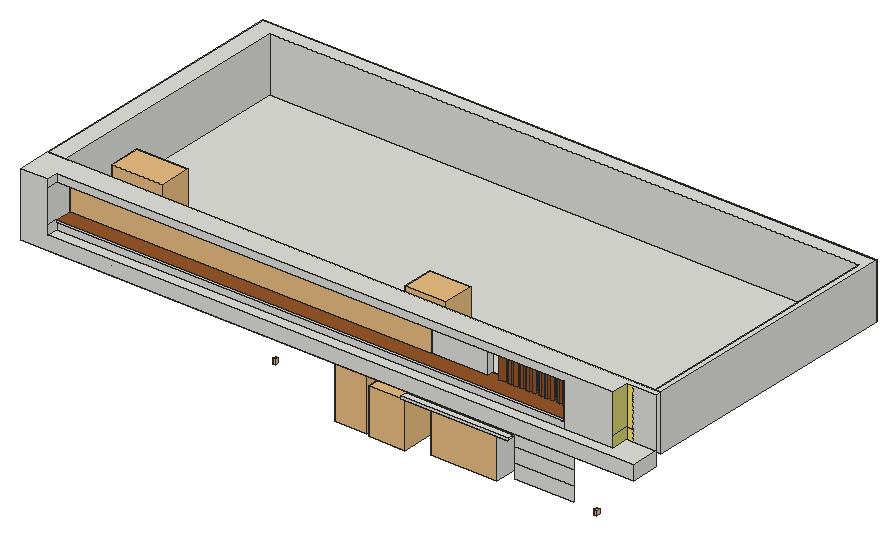
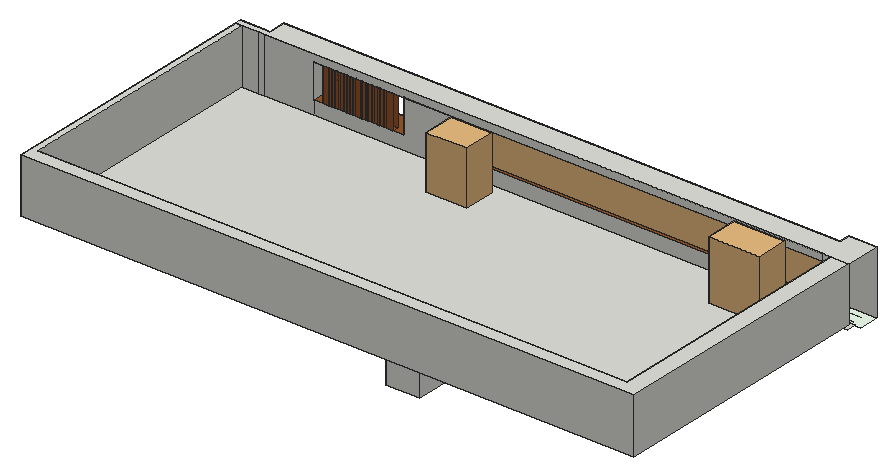
# SketchUp Ruby script. Lengths in inches.
U = 1.inch
M = Sketchup.active_model
def pt(a) = Geom::Point3d.new(a.map { |v| v * U })
def face(e, loops, mat)
  f = e.add_face(loops[0].map { |a| pt(a) })
  loops[1..].each { |l| e.add_face(l.map { |a| pt(a) }).erase! }
  f.material = f.back_material = mat if mat
  f
end
# faces: each face lists its corners as indices into pts; further lists are holes
def faces(e, pts, list, mat = nil) = list.each { |f| face(e, (f[0].is_a?(Array) ? f : [f]).map { |l| l.map { |i| pts[i] } }, mat) }
# xy, xz, yz: faces in a plane at the given z, y or x. An outline is a flat list of corners, or four numbers for a rectangle; further outlines are holes
def ring(l) = l.size == 4 ? [[l[0], l[1]], [l[2], l[1]], [l[2], l[3]], [l[0], l[3]]] : l.each_slice(2).to_a
def flat(e, list, mat, &to3) = list.each { |f| face(e, (f[0].is_a?(Array) ? f : [f]).map { |l| ring(l).map { |u, v| to3.(u, v) } }, mat) }
def xy(e, z, list, mat = nil) = flat(e, list, mat) { |x, y| [x, y, z] }
def xz(e, y, list, mat = nil) = flat(e, list, mat) { |x, z| [x, y, z] }
def yz(e, x, list, mat = nil) = flat(e, list, mat) { |y, z| [x, y, z] }
def lines(e, pts, list) = list.each { |a, b| e.add_line(pt(pts[a]), pt(pts[b])) }
# prism: a flat outline (further loops are holes) pulled along v
def prism(e, loops, v, mat = nil)
  f = face(e, loops, mat); d = Geom::Vector3d.new(v.map { |x| x * U })
  f.pushpull(f.normal.samedirection?(d) ? d.length : -d.length)
end
def box(e, o, s, mat = nil) = prism(e, [[o, [o[0] + s[0], o[1], o[2]], [o[0] + s[0], o[1] + s[1], o[2]], [o[0], o[1] + s[1], o[2]]]], [0, 0, s[2]], mat)
def at(x, y, z, deg = 0) = Geom::Transformation.translation(pt([x, y, z])) * Geom::Transformation.rotation(ORIGIN, Z_AXIS, deg.degrees)
def axes(o, x, y, z) = Geom::Transformation.new([*x, 0, *y, 0, *z, 0, *pt(o).to_a, 1])
def part(name) = M.definitions.add(name)
# library, detail: a bought-in or finely detailed component or shape, given as its bounding box
def library(name, o, s) = part(name).tap { |d| box(d.entities, o, s) }
def detail(e, o, s) = box(e.add_group.entities, o, s)
def put(e, d, t, mat = nil) = e.add_instance(d, t).tap { |i| i.material = mat if mat }
def group(e, t, mat = nil) = e.add_group.tap { |g| g.transformation = t; g.material = mat if mat }.entities
root = M.entities
M.materials.add("Emissive").color = [210, 207, 113]
M.materials.add("Generic").color = [255, 233, 107]
M.materials.add("[0066_Honeydew]").color = [240, 255, 240]
M.materials.add("[Wood Cherry Original]").color = [152, 86, 42]
M.materials.add("[Wood Veneer 01]").color = [120, 70, 37]
c1 = library("KentiaPalm",[-22.86,-14.31,0],[47.49,43.96,59.125])
c2 = library("cay+chuoi",[26.89,19.66,0.52],[41.96,45.65,69.71])
c3 = library("Group\#14",[0,0,0],[39.5,117.4375,51.17])
c4 = part("Group668\#1")
p = [[0,0,0],[0,0,-13.34],[-3.03,0,-13.34],[19.7,-23.5,0],[-19.7,-23.5,0],[19.7,23.5,0],
  [19.7,0,0],[-19.7,23.5,0],[3.03,0,-13.34],[-19.7,0,0],[0,0,-21.6]]
lines(c4.entities,p,[[0,1],[1,2],[3,4],[5,6],[7,5],[1,8],[9,0],[0,6],[8,10],[4,9],[6,3],[2,10],
  [9,7]])
c5 = part("Rectangle Light")
put(c5.entities,c4,at(0,0,0))
c6 = library("Lamp Wall Outdoor 94-02",[-1.89,-4.65,-3.17],[3.78,4.65,6.35])
c7 = part("Copyright 2018, ")
xy(c7.entities,0.05,[[[19.06,0,19.06,9.82,21.3125,9.82,22.13,9.76,22.85,9.6,23.48,9.33,24,8.95,24.43,8.48,24.73,7.92,24.91,7.28,24.97,6.54,24.91,5.85,24.74,5.21,24.46,4.64,24.0625,4.14,23.58,3.73,23.03,3.4375,22.42,3.26,21.75,3.2,21.1,3.27,20.375,3.48,20.375,0],[21.62,4.3125,22.05,4.35,22.4375,4.47,22.79,4.66,23.09,4.94,23.34,5.28,23.52,5.66,23.63,6.09,23.67,6.56,23.6,7.16,23.4,7.68,23.08,8.1,22.66,8.39,22.08,8.56,21.28,8.61,20.375,8.61,20.375,4.61,20.98,4.39]],[25.77,0,27.98,4.71,25.47,9.82,26.9375,9.82,28.69,6.14,30.375,9.82,31.82,9.82,27.21,0],[[43.77,0,43.11,0.03,42.52,0.14,41.99,0.3125,41.54,0.55,41.18,0.86,40.92,1.2,40.77,1.6,40.71,2.04,40.82,2.64,41.12,3.13,41.63,3.5,42.35,3.75,41.86,4.16,41.74,4.37,41.7,4.57,41.77,4.87,41.98,5.14,42.3,5.36,42.73,5.51,42.1,5.88,41.65,6.34,41.38,6.91,41.29,7.57,41.34,8.0625,41.48,8.5,41.72,8.88,42.05,9.21,42.47,9.48,42.95,9.67,43.5,9.78,44.13,9.82,46.81,9.82,46.81,8.8125,45.49,8.8125,46.02,8.11,46.13,7.77,46.17,7.38,46.1,6.875,45.88,6.38,45.55,5.94,45.13,5.625,44.53,5.39,43.64,5.21,43.09,5.03,42.96,4.89,42.91,4.71,42.98,4.5,43.18,4.34,44.17,4.04,45.71,3.625,46.33,3.2,46.67,2.67,46.79,2.03,46.74,1.59,46.59,1.2,46.33,0.85,45.97,0.55,45.52,0.31,45.01,0.14,44.42,0.03],[43.74,1.02,44.5,1.09,45.0625,1.28,45.42,1.58,45.53,1.99,45.5,2.2,45.39,2.4,44.94,2.72,44.26,2.9375,43.41,3.01,42.82,2.94,42.34,2.73,42.03,2.42,41.93,2.03,42.04,1.59,42.38,1.28,42.95,1.09],[43.72,6.34,44.22,6.42,44.63,6.67,44.91,7.05,45,7.51,44.9,7.98,44.63,8.36,44.22,8.61,43.71,8.7,43.23,8.61,42.82,8.35,42.54,7.96,42.45,7.5,42.54,7.04,42.8125,6.67,43.22,6.42]],[180.16,0,182.36,4.71,179.85,9.82,181.32,9.82,183.07,6.14,184.75,9.82,186.2,9.82,181.59,0],[[219.8,0,219.13,0.03,218.54,0.14,218.02,0.3125,217.57,0.55,217.21,0.86,216.95,1.2,216.79,1.6,216.74,2.04,216.84,2.64,217.15,3.13,217.66,3.5,218.375,3.75,217.89,4.16,217.77,4.37,217.72,4.57,217.79,4.87,218,5.14,218.33,5.36,218.76,5.51,218.13,5.88,217.68,6.34,217.41,6.91,217.32,7.57,217.37,8.0625,217.51,8.5,217.75,8.88,218.08,9.21,218.5,9.48,218.98,9.67,219.53,9.78,220.16,9.82,222.83,9.82,222.83,8.8125,221.52,8.8125,222.05,8.11,222.16,7.77,222.2,7.38,222.125,6.875,221.91,6.38,221.58,5.94,221.16,5.625,220.5625,5.39,219.67,5.21,219.12,5.03,218.99,4.89,218.94,4.71,219.01,4.5,219.21,4.34,220.2,4.04,221.73,3.625,222.35,3.2,222.7,2.67,222.82,2.03,222.77,1.59,222.61,1.2,222.36,0.85,222,0.55,221.55,0.31,221.03,0.14,220.45,0.03],[219.77,1.02,220.53,1.09,221.09,1.28,221.44,1.58,221.5625,1.99,221.52,2.2,221.41,2.4,220.97,2.72,220.29,2.9375,219.43,3.01,218.84,2.94,218.37,2.73,218.0625,2.42,217.96,2.03,218.07,1.59,218.41,1.28,218.98,1.09],[219.75,6.34,220.25,6.42,220.66,6.67,220.93,7.05,221.02,7.51,220.93,7.98,220.66,8.36,220.24,8.61,219.74,8.7,219.25,8.61,218.85,8.35,218.57,7.96,218.48,7.5,218.57,7.04,218.84,6.67,219.25,6.42]],
  [92.62,1.6,92.62,1.87,92.89,2.17,93.07,2.48,93.22,3.3125,92.89,3.45,92.65,3.66,92.51,3.92,92.47,4.24,92.53,4.6,92.72,4.9,93.01,5.11,93.34,5.18,93.73,5.08,94.04,4.8,94.25,4.36,94.32,3.82,94.2,3.09,93.87,2.45,93.33,1.9375],[6.01,3.2,5.21,3.24,4.48,3.37,3.81,3.58,3.2,3.87,2.66,4.23,2.17,4.66,1.74,5.14,1.38,5.7,1.08,6.29,0.875,6.91,0.75,7.55,0.71,8.22,0.8,9.25,1.09,10.2,1.57,11.07,2.24,11.84,3.06,12.49,3.96,12.95,4.95,13.22,6.04,13.3125,6.83,13.26,7.68,13.11,8.5625,12.86,9.49,12.5,9.49,10.98,8.63,11.42,7.78,11.72,6.9375,11.91,6.11,11.97,5.29,11.9,4.55,11.7,3.89,11.37,3.29,10.9,2.8,10.33,2.45,9.7,2.24,8.99,2.17,8.22,2.24,7.44,2.45,6.74,2.79,6.11,3.27,5.55,3.86,5.09,4.53,4.76,5.27,4.57,6.09,4.5,6.98,4.57,7.87,4.78,8.74,5.12,9.6,5.6,9.6,4.05,8.79,3.68,7.92,3.41,6.99,3.25],[[14.21,3.2,13.51,3.26,12.87,3.4375,12.29,3.73,11.77,4.14,11.34,4.65,11.03,5.21,10.85,5.82,10.78,6.5,10.85,7.1875,11.03,7.81,11.34,8.375,11.78,8.88,12.31,9.3,12.9,9.59,13.55,9.77,14.27,9.83,14.98,9.77,15.63,9.59,16.21,9.29,16.73,8.87,17.16,8.36,17.47,7.79,17.66,7.16,17.72,6.47,17.66,5.79,17.47,5.18,17.16,4.625,16.72,4.13,16.19,3.72,15.6,3.43,14.9375,3.26],[14.25,4.4,14.71,4.44,15.12,4.55,15.48,4.74,15.81,5,16.07,5.32,16.26,5.68,16.37,6.08,16.41,6.53,16.37,6.97,16.25,7.375,16.06,7.74,15.78,8.0625,15.45,8.33,15.07,8.52,14.65,8.63,14.2,8.67,13.76,8.63,13.36,8.52,13,8.33,12.68,8.0625,12.42,7.74,12.23,7.37,12.12,6.97,12.08,6.52,12.12,6.07,12.24,5.67,12.43,5.31,12.69,4.99,13.02,4.73,13.39,4.55,13.8,4.44]],[57.3125,3.2,56.51,3.33,55.84,3.72,55.54,4.07,55.34,4.58,55.26,5.77,55.26,8.66,54.13,8.66,54.13,8.78,56.54,11.16,56.54,9.82,58.6,9.82,58.6,8.66,56.54,8.66,56.54,5.48,56.6,4.99,56.78,4.64,57.06,4.43,57.47,4.36,58.18,4.48,58.93,4.82,58.93,3.62,58.16,3.31],[[88.3125,3.2,87.67,3.25,87.08,3.41,86.54,3.66,86.06,4.02,85.66,4.45,85.37,4.93,85.2,5.46,85.14,6.04,85.23,6.75,85.49,7.37,85.93,7.91,86.54,8.36,86,8.86,85.64,9.37,85.4375,9.91,85.37,10.54,85.43,11.1,85.59,11.61,85.86,12.08,86.24,12.51,86.7,12.86,87.21,13.11,87.76,13.26,88.37,13.3125,88.96,13.26,89.51,13.11,90.01,12.86,90.46,12.51,90.83,12.09,91.09,11.62,91.25,11.1,91.31,10.54,91.23,9.91,91,9.33,90.62,8.82,90.08,8.36,90.68,7.91,91.11,7.38,91.36,6.75,91.45,6.02,91.39,5.4375,91.23,4.91,90.95,4.43,90.56,4,90.08,3.65,89.55,3.4,88.96,3.25],[88.33,4.54,89,4.64,89.54,4.94,89.9,5.39,90.02,5.96,90.02,6.11,89.9,6.72,89.54,7.21,88.98,7.53,88.28,7.64,87.6,7.53,87.05,7.21,86.69,6.71,86.57,6.09,86.69,5.47,87.06,4.98,87.62,4.65],[88.35,9.02,88.95,9.125,89.45,9.45,89.79,9.93,89.9,10.49,89.79,11.08,89.46,11.55,88.96,11.87,88.34,11.97,87.72,11.87,87.22,11.5625,86.89,11.09,86.78,10.51,86.89,9.9375,87.24,9.46,87.75,9.13]],
  [[113.29,3.2,112.92,3.24,112.64,3.36,112.43,3.57,112.32,3.85,111.9,3.57,111.47,3.375,111.03,3.26,110.57,3.22,109.95,3.33,109.44,3.66,109.1,4.17,108.99,4.79,109.1,5.375,109.43,5.89,109.97,6.32,110.6875,6.66,112.33,7.22,112.33,7.57,112.26,8.08,112.04,8.45,111.67,8.67,111.16,8.74,110.64,8.67,110.12,8.47,109.61,8.13,109.11,7.65,109.11,9.06,109.53,9.45,110.02,9.72,110.6,9.89,111.27,9.94,111.77,9.91,112.21,9.81,112.61,9.63,112.95,9.39,113.34,8.92,113.55,8.34,113.6,7.22,113.6,4.46,113.65,4.21,113.82,4.13,114.12,4.21,114.55,4.47,114.55,3.6875,113.85,3.3],[111.19,4.1,111.79,4.22,112.33,4.6,112.33,6.53,111.47,6.2,110.91,5.9375,110.54,5.67,110.34,5.375,110.27,5.01,110.33,4.64,110.53,4.35,110.82,4.16]],[121.02,3.2,120.43,3.28,119.88,3.51,119.43,3.87,119.1,4.34,118.9,5.04,118.83,6.09,118.83,9.82,120.12,9.82,120.12,6.11,120.19,5.24,120.41,4.68,120.82,4.38,121.44,4.28,121.88,4.33,122.29,4.5,122.66,4.78,123,5.17,123,9.82,124.29,9.82,124.29,3.3125,123,3.3125,123,4.15,122.5625,3.75,122.07,3.45,121.54,3.26],[[156.36,3.2,155.99,3.24,155.7,3.36,155.5,3.57,155.39,3.85,154.97,3.57,154.54,3.375,154.1,3.26,153.64,3.22,153.02,3.33,152.51,3.66,152.17,4.17,152.06,4.79,152.17,5.375,152.5,5.89,153.03,6.32,153.75,6.66,155.4,7.22,155.4,7.57,155.33,8.08,155.11,8.45,154.74,8.67,154.23,8.74,153.7,8.67,153.1875,8.47,152.68,8.13,152.18,7.65,152.18,9.06,152.59,9.45,153.09,9.72,153.67,9.89,154.33,9.94,154.83,9.91,155.28,9.81,155.68,9.63,156.02,9.39,156.4,8.92,156.62,8.34,156.66,7.22,156.66,4.46,156.72,4.21,156.89,4.13,157.1875,4.21,157.62,4.47,157.62,3.6875,156.92,3.3],[154.26,4.1,154.85,4.22,155.4,4.6,155.4,6.53,154.54,6.2,153.98,5.9375,153.61,5.67,153.4,5.375,153.34,5.01,153.4,4.64,153.59,4.35,153.89,4.16]],[161.74,3.2,161.01,3.26,160.37,3.43,159.8,3.71,159.3,4.11,158.91,4.6,158.62,5.16,158.45,5.81,158.4,6.53,158.45,7.26,158.62,7.92,158.89,8.5,159.28,9,159.76,9.41,160.3,9.71,160.92,9.88,161.6,9.94,162.51,9.85,163.49,9.49,163.49,8.12,162.55,8.59,161.68,8.74,161.27,8.7,160.89,8.59,160.55,8.4,160.25,8.13,160.01,7.8,159.84,7.4375,159.73,7.02,159.7,6.57,159.73,6.1,159.85,5.68,160.04,5.31,160.3,4.99,160.63,4.73,161.01,4.55,161.44,4.4375,161.93,4.4,162.73,4.51,163.63,4.83,163.63,3.5625,162.67,3.29],[[178.37,3.2,178,3.24,177.71,3.36,177.51,3.57,177.39,3.85,176.98,3.57,176.55,3.375,176.1,3.26,175.65,3.22,175.02,3.33,174.52,3.66,174.18,4.17,174.0625,4.79,174.17,5.375,174.51,5.89,175.04,6.32,175.76,6.66,177.41,7.22,177.41,7.57,177.33,8.08,177.11,8.45,176.75,8.67,176.23,8.74,175.71,8.67,175.19,8.47,174.6875,8.13,174.18,7.65,174.18,9.06,174.6,9.45,175.1,9.72,175.68,9.89,176.34,9.94,176.84,9.91,177.29,9.81,177.68,9.63,178.03,9.39,178.41,8.92,178.625,8.34,178.67,7.22,178.67,4.46,178.73,4.21,178.9,4.13,179.2,4.21,179.625,4.47,179.625,3.6875,178.92,3.3],[176.27,4.1,176.86,4.22,177.41,4.6,177.41,6.53,176.54,6.2,175.98,5.9375,175.61,5.67,175.41,5.375,175.34,5.01,175.41,4.64,175.6,4.35,175.9,4.16]],
  [210.76,3.2,209.73,3.33,208.59,3.78,208.59,5.17,209.71,4.55,210.23,4.37,210.66,4.3125,211.04,4.36,211.36,4.51,211.57,4.73,211.65,4.98,211.6,5.24,211.46,5.45,210.65,5.99,209.62,6.64,209.02,7.18,208.73,7.69,208.64,8.25,208.67,8.6,208.78,8.93,208.96,9.22,209.22,9.47,209.89,9.83,210.72,9.94,211.6875,9.81,212.68,9.41,212.68,8.13,211.64,8.65,210.81,8.83,210.47,8.79,210.2,8.67,210.03,8.48,209.97,8.25,210.02,8.03,210.18,7.82,210.91,7.32,211.37,7.06,212.08,6.59,212.59,6.09,212.89,5.57,213,5.02,212.96,4.64,212.84,4.3,212.64,3.99,212.37,3.71,212.04,3.49,211.66,3.33],[[73.82,3.22,73.14,3.3,72.53,3.56,71.99,3.99,71.52,4.59,71.14,5.34,70.87,6.2,70.7,7.17,70.65,8.25,70.71,9.32,70.875,10.29,71.16,11.15,71.55,11.9,72.03,12.52,72.58,12.96,73.2,13.23,73.88,13.3125,74.53,13.23,75.12,12.96,75.65,12.51,76.125,11.89,76.51,11.13,76.79,10.27,76.96,9.32,77.01,8.28,76.96,7.2,76.79,6.24,76.51,5.38,76.125,4.62,75.65,4.01,75.11,3.57,74.5,3.3],[73.81,4.52,74.2,4.58,74.54,4.77,74.84,5.08,75.1,5.51,75.31,6.06,75.46,6.6875,75.58,8.22,75.46,9.76,75.32,10.4,75.12,10.95,74.87,11.4,74.59,11.72,74.26,11.91,73.89,11.97,73.82,11.97,73.4375,11.91,73.09,11.72,72.79,11.41,72.53,10.97,72.32,10.43,72.18,9.79,72.06,8.26,72.17,6.7,72.32,6.06,72.52,5.51,72.78,5.08,73.08,4.77,73.42,4.58]],[[204.86,3.22,203.89,3.33,203.125,3.66,202.53,4.18,202.06,4.86,201.76,5.67,201.66,6.6,201.71,7.31,201.87,7.95,202.13,8.51,202.5,9.01,202.95,9.42,203.47,9.71,204.05,9.89,204.6875,9.94,205.3,9.89,205.85,9.72,206.33,9.43,206.75,9.04,207.09,8.55,207.33,7.98,207.47,7.34,207.52,6.61,207.52,6.45,202.95,6.45,203.13,5.61,203.32,5.27,203.57,4.97,203.88,4.73,204.23,4.55,205.06,4.42,205.68,4.47,206.28,4.61,206.86,4.86,207.41,5.21,207.41,3.95,206.82,3.61,206.23,3.39,205.6,3.26],[202.98,7.22,206.25,7.22,206.11,7.9,205.79,8.41,205.31,8.72,204.6875,8.83,204.06,8.72,203.55,8.41,203.1875,7.9]],[32.81,3.3125,32.81,9.82,34.1,9.82,34.1,8.33,34.17,8.4375,34.64,9.1,35.1,9.57,35.57,9.85,36.04,9.94,36.4,9.9,36.78,9.76,37.55,9.21,36.875,8.08,36.23,8.55,35.63,8.71,35.33,8.68,35.05,8.57,34.55,8.12,34.21,7.47,34.1,6.71,34.1,3.3125],[38.48,3.3125,39.77,9.82],
  [47.77,3.3125,47.77,13.1875,49.06,13.1875,49.06,8.96,49.49,9.39,49.96,9.7,50.49,9.88,51.06,9.94,51.68,9.86,52.23,9.62,52.68,9.23,52.99,8.72,53.18,8.01,53.24,7.02,53.24,3.3125,51.96,3.3125,51.96,7.34,51.87,7.98,51.61,8.48,51.2,8.81,50.6875,8.92,50.27,8.86,49.89,8.7,49.49,8.41,49.06,7.97,49.06,3.3125],[63.46,3.3125,63.46,3.41,64.06,4.11,66.27,7.04,66.95,8.09,67.35,8.86,67.53,9.47,67.6,10.07,67.48,10.82,67.125,11.41,66.57,11.79,65.87,11.92,65.28,11.83,64.7,11.57,64.15,11.14,63.66,10.58,63.66,12.375,64.24,12.79,64.83,13.08,65.43,13.26,66.04,13.3125,66.65,13.26,67.21,13.1,67.72,12.83,68.17,12.45,68.53,11.99,68.79,11.47,68.95,10.9,69,10.26,68.95,9.65,68.8,8.99,68.51,8.27,68.06,7.4375,67.34,6.4,66.26,5.04,65.95,4.68,69.71,4.68,69.71,3.3125],[80.37,3.3125,81.78,13.1875],[100.21,3.3125,100.21,13.1875,101.625,13.1875,101.625,8.67,105.78,13.1875,107.55,13.1875,103.27,8.5,108.6,3.3125,106.67,3.3125,101.625,8.19,101.625,3.3125],[115.72,3.3125,117,13.1875],
  [126.04,3.3125,126.04,9.82,127.33,9.82,127.33,8.96,127.82,9.39,128.3,9.7,128.78,9.88,129.25,9.94,129.83,9.87,130.35,9.65,130.79,9.28,131.17,8.77,131.6875,9.29,132.22,9.66,132.77,9.88,133.32,9.96,133.77,9.91,134.18,9.78,134.55,9.57,134.88,9.27,135.15,8.875,135.34,8.39,135.45,7.82,135.49,7.15,135.49,3.3125,134.2,3.3125,134.2,7.17,134.12,7.88,133.87,8.41,133.47,8.73,132.92,8.84,132.53,8.79,132.15,8.64,131.78,8.39,131.43,8.04,131.43,3.3125,130.13,3.3125,130.13,6.93,130.0625,7.85,129.84,8.44,129.67,8.63,129.45,8.76,128.83,8.87,128.45,8.82,128.1,8.6875,127.74,8.43,127.33,8.04,127.33,3.3125],[141.43,3.3125,141.43,13.1875,142.77,13.1875,146.05,9.13,149.31,13.1875,150.63,13.1875,150.63,3.3125,149.21,3.3125,149.21,11,146.17,7.18,145.91,7.18,142.84,11,142.84,3.3125],[165.29,3.3125,165.29,13.1875,166.7,13.1875,166.7,8.67,170.86,13.1875,172.62,13.1875,168.34,8.5,173.67,3.3125,171.75,3.3125,166.7,8.19,166.7,3.3125],[214.51,3.3125,215.8,9.82],[223.8,3.3125,223.8,9.82,225.12,9.82,225.12,8.99,225.5625,9.41,226.04,9.7,226.54,9.88,227.07,9.94,227.66,9.86,228.2,9.63,228.67,9.26,229,8.77,229.2,8.06,229.27,7.03,229.27,3.3125,227.99,3.3125,227.99,7.02,227.91,7.87,227.68,8.44,227.28,8.76,226.66,8.87,226.23,8.8125,225.82,8.64,225.45,8.36,225.12,7.96,225.12,3.3125],
  [[191.3125,3.33,191.3125,13.1875,194.64,13.1875,195.6,13.15,196.45,13.04,197.19,12.85,197.83,12.58,198.39,12.25,198.88,11.84,199.32,11.36,199.7,10.81,200,10.21,200.22,9.58,200.35,8.93,200.39,8.25,200.29,7.28,200.01,6.35,199.54,5.5,198.92,4.76,198.14,4.14,197.24,3.7,196.22,3.4,194.4375,3.33],[192.73,4.59,194.54,4.59,195.48,4.62,196.18,4.73,197.16,5.1,197.88,5.65,198.34,6.21,198.66,6.85,198.86,7.55,198.93,8.33,198.86,9.08,198.66,9.77,198.32,10.38,197.85,10.92,197.43,11.26,196.94,11.53,195.97,11.85,194.49,11.93,192.73,11.93]],[39.12,11.03,38.84,11.09,38.59,11.26,38.42,11.51,38.37,11.8,38.42,12.08,38.59,12.32,38.84,12.49,39.12,12.55,39.41,12.5,39.66,12.33,39.83,12.09,39.89,11.8,39.83,11.51,39.66,11.26,39.41,11.09],[215.14,11.03,214.87,11.09,214.62,11.26,214.45,11.51,214.4,11.8,214.45,12.08,214.62,12.32,214.87,12.49,215.14,12.55,215.44,12.5,215.6875,12.33,215.86,12.09,215.92,11.8,215.86,11.51,215.6875,11.26,215.44,11.09]])
c8 = library("Spot Light",[-8.21,-8.21,-2.75],[16.42,16.42,2.75])
c9 = library("Tlon Light 1950 Ceiling 152 010",[-38.39,-38.39,-3.78],[76.78,76.78,3.41])
c10 = library("plant",[-21.34,-27.21,-0.38],[41.91,41.15,38.97])
c11 = library("Glass Railings(black Handrails)",[-57.04,-132.55,0],[169.29,2.52,28.17])
xy(root,382.92,[[1005.21,916.1875,1091.46,1037.5]])
xy(root,403.73,[[834.07,1080.1875,878.82,1086.1875],[834.07,1080.1875,878.82,1204.875]])
xy(root,405.89,[[836.23,1080.1875,876.66,1081.4375],[836.23,1084.9375,876.66,1086.1875]])
xy(root,406.52,[[836.87,1081.4375,876.02,1082.6875],[836.87,1082.6875,876.02,1083.6875],[836.87,1083.6875,876.02,1084.9375]])
xy(root,407.05,[[837.4,1082.6875,875.5,1082.79],[837.4,1082.79,875.5,1083.59],[837.4,1083.59,875.5,1083.6875]])
xy(root,440.98,[[1005.21,916.1875,1091.46,1037.5]])
xy(root,441.7,[[973.0625,907.15,1112.75,916.1875]])
xy(root,444.51,[[973.0625,907.15,1112.75,916.1875]])
xy(root,445.15,[[837.4,1082.6875,875.5,1082.79],[837.4,1082.79,875.5,1083.59],[837.4,1083.59,875.5,1083.6875]])
xy(root,445.68,[[836.87,1081.4375,876.02,1082.6875],[836.87,1082.6875,876.02,1083.6875],[836.87,1083.6875,876.02,1084.9375]])
xy(root,446.32,[[836.23,1080.1875,876.66,1081.4375],[836.23,1084.9375,876.66,1086.1875]])
xy(root,448.48,[[834.07,1080.1875,878.82,1086.1875],[834.07,1080.1875,878.82,1204.875]])
xy(root,454.24,[[624.25,1080.1875,714.02,1211.5]])
xy(root,457.58,[[973.0625,998.1875,995.625,1042.875]])
xy(root,469.7,[[973.0625,907.15,1112.75,916.1875]])
xy(root,472.51,[[505.625,904.1875,616.25,916.1875]])
xy(root,472.51,[[497.625,879.3125,624.25,904.1875],[973.0625,879.3125,973.0625,907.15,1112.75,907.15,1112.75,919.75,1189.1875,919.75,1189.1875,908.4375,1197.1875,908.4375,1197.1875,916.1875,1299.8125,916.1875,1299.8125,879.3125]],"[0066_Honeydew]")
xy(root,472.51,[[[624.25,879.3125,973.0625,1080.1875],[782.66,915.1875,785.84,915.1875,785.84,916.1875,817.03,916.1875,817.03,915.1875,820.03,915.1875,820.03,920.9375,782.66,920.9375]]],"[Wood Veneer 01]")
xy(root,484.51,[[497.625,924.1875,497.625,1276.1875,1299.8125,1276.1875,1299.8125,924.1875,1291.8125,924.1875,1291.8125,1258.125,520.65,1258.125,520.65,924.1875],[520.65,924.1875,1291.8125,1258.125]])
xy(root,491.26,[[533.4375,879.3125,1299.8125,879.3125,1299.8125,916.1875,1261.34,916.1875,1261.34,893.8125,533.4375,893.8125]])
xy(root,500.61,[[533.4375,893.01,1197.1875,893.8125]])
xy(root,502.61,[[1105.94,916.1875,1110.61,924.1875],[1121.91,916.1875,1126.57,924.1875],[1129.89,916.1875,1134.56,924.1875],[1145.85,916.1875,1150.52,924.1875],[1153.83,916.1875,1158.5,924.1875],
  [1169.79,916.1875,1174.46,924.1875],[1177.77,916.1875,1185.76,924.1875]])
xy(root,502.61,[[533.4375,893.01,1197.1875,893.01,1197.1875,924.1875,1185.76,924.1875,1185.76,916.1875,1177.77,916.1875,1177.77,924.1875,1174.46,924.1875,1174.46,916.1875,1169.79,916.1875,1169.79,924.1875,1166.48,924.1875,1166.48,916.1875,1161.8125,916.1875,1161.8125,924.1875,1158.5,924.1875,1158.5,916.1875,1153.83,916.1875,1153.83,924.1875,1150.52,924.1875,1150.52,916.1875,1145.85,916.1875,1145.85,924.1875,1142.54,924.1875,1142.54,916.1875,1137.87,916.1875,1137.87,924.1875,1134.56,924.1875,1134.56,916.1875,1129.89,916.1875,1129.89,924.1875,1126.57,924.1875,1126.57,916.1875,1121.91,916.1875,1121.91,924.1875,1118.59,924.1875,1118.59,916.1875,1113.92,916.1875,1113.92,924.1875,1110.61,924.1875,1110.61,916.1875,1105.94,916.1875,1105.94,924.1875,1102.63,924.1875,1102.63,916.1875,1094.65,916.1875,1094.65,924.1875,1079.59,924.1875,1079.59,916.1875,1005.75,916.1875,1005.75,924.1875,533.4375,924.1875],[1094.65,916.1875,1102.63,924.1875],[1113.92,916.1875,1118.59,924.1875],[1137.87,916.1875,1142.54,924.1875],[1161.8125,916.1875,1166.48,924.1875]],"[Wood Cherry Original]")
xy(root,546.59,[[533.4375,893.8125,533.4375,924.1875,1105.94,924.1875,1105.94,916.1875,1110.61,916.1875,1110.61,924.1875,1121.91,924.1875,1121.91,916.1875,1126.57,916.1875,1126.57,924.1875,1129.89,924.1875,1129.89,916.1875,1134.56,916.1875,1134.56,924.1875,1145.85,924.1875,1145.85,916.1875,1150.52,916.1875,1150.52,924.1875,1153.83,924.1875,1153.83,916.1875,1158.5,916.1875,1158.5,924.1875,1169.79,924.1875,1169.79,916.1875,1174.46,916.1875,1174.46,924.1875,1177.77,924.1875,1177.77,916.1875,1185.76,916.1875,1185.76,924.1875,1197.1875,924.1875,1197.1875,893.8125,1079.59,893.8125,1079.59,916.1875,1005.75,916.1875,1005.75,893.8125]])
xy(root,546.8,[[1005.75,893.8125,1079.59,916.1875],[1005.75,916.1875,1079.59,924.1875]])
xy(root,556.51,[[497.625,879.3125,533.4375,879.3125,533.4375,893.8125,1261.34,893.8125,1261.34,916.1875,1299.8125,916.1875,1299.8125,924.1875,497.625,924.1875],[497.625,924.1875,520.65,924.1875,520.65,1258.125,1291.8125,1258.125,1291.8125,924.1875,1299.8125,924.1875,1299.8125,1276.1875,497.625,1276.1875]])
xz(root,879.3125,[[497.625,472.51,1299.8125,472.51,1299.8125,491.26,533.4375,491.26,533.4375,556.51,497.625,556.51]])
xz(root,893.01,[[533.4375,500.61,1197.1875,502.61]])
xz(root,893.8125,[[1197.1875,491.26,1261.34,491.26,1261.34,556.51,533.4375,556.51,533.4375,546.59,1005.75,546.59,1005.75,546.8,1079.59,546.8,1079.59,546.59,1197.1875,546.59],[533.4375,491.26,1197.1875,500.61]])
xz(root,907.15,[[973.0625,441.7,1112.75,444.51],[973.0625,469.7,1112.75,472.51]])
xz(root,916.1875,[[973.0625,444.51,1112.75,469.7],[1269.34,491.26,1299.8125,556.51],[1005.75,502.61,1079.59,546.59],[1005.75,546.59,1079.59,546.8]])
xz(root,916.1875,[[1261.34,491.26,1269.34,505.69],[1261.34,505.69,1269.34,556.51]],"Generic")
xz(root,916.1875,[[1094.65,502.61,1102.63,547.68],[1105.94,502.61,1110.61,546.59],[1113.92,502.61,1118.59,547.3],[1121.91,502.61,1126.57,546.59],[1129.89,502.61,1134.56,546.59],
  [1137.87,502.61,1142.54,548.55],[1145.85,502.61,1150.52,546.59],[1153.83,502.61,1158.5,546.59],[1161.8125,502.61,1166.48,548.36],[1169.79,502.61,1174.46,546.59],
  [1177.77,502.61,1185.76,546.59]],"[Wood Cherry Original]")
xz(root,919.75,[[1112.75,391.51,1189.1875,410.11],[1112.75,410.11,1189.1875,428.71],[1112.75,428.71,1189.1875,447.31],[1112.75,447.31,1189.1875,472.51]])
xz(root,924.1875,[[497.625,484.51,520.65,556.51],[520.65,484.51,520.65,556.51,533.4375,556.51,533.4375,502.61,1005.75,502.61,1005.75,546.59,1079.59,546.59,1079.59,502.61,1197.1875,502.61,1197.1875,484.51],[1197.1875,484.51,1197.1875,546.59,1079.59,546.59,1079.59,546.8,1005.75,546.8,1005.75,546.59,533.4375,546.59,533.4375,556.51,1261.34,556.51,1261.34,484.51],[1261.34,484.51,1269.34,556.51],[1269.34,484.51,1291.8125,556.51],
  [1291.8125,484.51,1299.8125,556.51],[1005.75,546.59,1079.59,546.8]])
xz(root,924.1875,[[1094.65,502.61,1102.63,546.59],[1102.63,502.61,1105.94,546.59],[1105.94,502.61,1110.61,546.59],[1110.61,502.61,1113.92,546.59],[1113.92,502.61,1118.59,546.59],
  [1118.59,502.61,1121.91,546.59],[1121.91,502.61,1126.57,546.59],[1126.57,502.61,1129.89,546.59],[1129.89,502.61,1134.56,546.59],[1134.56,502.61,1137.87,546.59],
  [1137.87,502.61,1142.54,546.59],[1142.54,502.61,1145.85,546.59],[1145.85,502.61,1150.52,546.59],[1150.52,502.61,1153.83,546.59],[1153.83,502.61,1158.5,546.59],
  [1158.5,502.61,1161.8125,546.59],[1161.8125,502.61,1166.48,546.59],[1166.48,502.61,1169.79,546.59],[1169.79,502.61,1174.46,546.59],[1174.46,502.61,1177.77,546.59],
  [1177.77,502.61,1185.76,546.59]],"[Wood Cherry Original]")
xz(root,1037.5,[[1005.21,382.92,1091.46,440.98]])
xz(root,1080.1875,[[[834.07,403.73,878.82,448.48],[836.23,405.89,876.66,446.32]]])
xz(root,1081.4375,[[[836.23,405.89,876.66,446.32],[836.87,406.52,876.02,445.68]]])
xz(root,1082.6875,[[[836.87,406.52,876.02,445.68],[837.4,407.05,875.5,445.15]]])
xz(root,1082.79,[[837.4,407.05,875.5,445.15]])
xz(root,1083.59,[[837.4,407.05,875.5,445.15]])
xz(root,1083.6875,[[[836.87,406.52,876.02,445.68],[837.4,407.05,875.5,445.15]]])
xz(root,1084.9375,[[[836.23,405.89,876.66,446.32],[836.87,406.52,876.02,445.68]]])
xz(root,1086.1875,[[[834.07,403.73,878.82,448.48],[836.23,405.89,876.66,446.32]]])
xz(root,1204.875,[[834.07,403.73,878.82,448.48]])
xz(root,1258.125,[[520.65,484.51,1291.8125,556.51]])
xz(root,1276.1875,[[497.625,484.51,1299.8125,556.51]])
yz(root,497.625,[[924.1875,484.51,1276.1875,556.51]])
yz(root,520.65,[[924.1875,484.51,1258.125,556.51]])
yz(root,533.4375,[[879.3125,491.26,893.8125,491.26,893.8125,500.61,893.01,500.61,893.01,502.61,879.3125,502.61],[879.3125,502.61,924.1875,546.59],[879.3125,546.59,893.8125,556.51]])
yz(root,834.07,[[1080.1875,403.73,1086.1875,448.48],[1080.1875,403.73,1204.875,448.48]])
yz(root,836.23,[[1080.1875,405.89,1081.4375,446.32],[1084.9375,405.89,1086.1875,446.32]])
yz(root,836.87,[[1081.4375,406.52,1082.6875,445.68],[1082.6875,406.52,1083.6875,445.68],[1083.6875,406.52,1084.9375,445.68]])
yz(root,837.4,[[1082.6875,407.05,1082.79,445.15],[1082.79,407.05,1083.59,445.15],[1083.59,407.05,1083.6875,445.15]])
yz(root,875.5,[[1082.6875,407.05,1082.79,445.15],[1082.79,407.05,1083.59,445.15],[1083.59,407.05,1083.6875,445.15]])
yz(root,876.02,[[1081.4375,406.52,1082.6875,445.68],[1082.6875,406.52,1083.6875,445.68],[1083.6875,406.52,1084.9375,445.68]])
yz(root,876.66,[[1080.1875,405.89,1081.4375,446.32],[1084.9375,405.89,1086.1875,446.32]])
yz(root,878.82,[[1080.1875,403.73,1086.1875,448.48],[1080.1875,403.73,1204.875,448.48]])
yz(root,1005.21,[[916.1875,382.92,1037.5,440.98]])
yz(root,1005.75,[[916.1875,502.61,924.1875,546.8],[893.8125,546.59,916.1875,546.8]])
yz(root,1079.59,[[916.1875,502.61,924.1875,546.8],[893.8125,546.59,916.1875,546.8]])
yz(root,1091.46,[[916.1875,382.92,1037.5,440.98]])
yz(root,1105.94,[[916.1875,502.61,924.1875,546.59]],"[Wood Cherry Original]")
yz(root,1110.61,[[916.1875,502.61,924.1875,546.59]],"[Wood Cherry Original]")
yz(root,1121.91,[[916.1875,502.61,924.1875,546.59]],"[Wood Cherry Original]")
yz(root,1126.57,[[916.1875,502.61,924.1875,546.59]],"[Wood Cherry Original]")
yz(root,1129.89,[[916.1875,502.61,924.1875,546.59]],"[Wood Cherry Original]")
yz(root,1134.56,[[916.1875,502.61,924.1875,546.59]],"[Wood Cherry Original]")
yz(root,1145.85,[[916.1875,502.61,924.1875,546.59]],"[Wood Cherry Original]")
yz(root,1150.52,[[916.1875,502.61,924.1875,546.59]],"[Wood Cherry Original]")
yz(root,1153.83,[[916.1875,502.61,924.1875,546.59]],"[Wood Cherry Original]")
yz(root,1158.5,[[916.1875,502.61,924.1875,546.59]],"[Wood Cherry Original]")
yz(root,1169.79,[[916.1875,502.61,924.1875,546.59]],"[Wood Cherry Original]")
yz(root,1174.46,[[916.1875,502.61,924.1875,546.59]],"[Wood Cherry Original]")
yz(root,1177.77,[[916.1875,502.61,924.1875,546.59]],"[Wood Cherry Original]")
yz(root,1185.76,[[916.1875,502.61,924.1875,546.59]],"[Wood Cherry Original]")
yz(root,1197.1875,[[893.01,500.61,893.8125,502.61],[893.8125,502.61,924.1875,546.59]])
yz(root,1261.34,[[893.8125,491.26,916.1875,505.69],[893.8125,505.69,916.1875,556.51]],"Emissive")
yz(root,1291.8125,[[924.1875,484.51,1258.125,556.51]])
yz(root,1299.8125,[[879.3125,472.51,916.1875,491.26],[924.1875,484.51,1276.1875,556.51]])
p = [[624.25,1080.1875,483.26],[714.02,1080.1875,483.26],[714.02,1080.1875,472.51],[497.625,916.1875,484.51],[616.25,916.1875,484.51],[616.25,916.1875,472.51],
  [616.25,904.1875,484.51],[497.625,904.1875,484.51],[616.25,879.3125,484.51],[1094.65,924.1875,547.68],[1094.65,916.1875,547.68],[1113.92,916.1875,547.3],
  [1113.92,924.1875,547.3],[1142.54,924.1875,548.55],[1142.54,916.1875,548.55],[1166.48,924.1875,548.36],[1166.48,916.1875,548.36]]
lines(root,p,[[0,1],[2,1],[3,4],[5,4],[4,6],[6,7],[6,8],[9,10],[11,12],[13,14],[15,16]])
put(root,c1,at(947.49,929.5,377.14))
put(root,c2,at(853.12,895.71,378.71))
put(root,c3,axes([1005.38,916.1875,382.92],[2.1792,0,0],[0,0.536,0],[0,0,1.13471]))
put(root,c5,axes([1050.32,1037.49,408.48],[1,0,0],[0,0,-1],[0,1,0]))
put(root,c6,at(1224.3125,916.1875,394.49))
put(root,c7,axes([840.86,1084.41,403.73],[0.13928,0,0],[0,-0.1494,0],[0,0,-0.93236]))
put(root,c6,at(803.67,916.1875,423.89))
put(root,c7,axes([872.05,1084.14,446.98],[-0.13928,0,0],[0,-0.1494,0],[0,0,0.93236]))
put(root,c8,axes([684.35,1134.96,454.25],[0.32,0,0],[0,0.32,0],[0,0,0.32]))
put(root,c9,axes([698.67,949.92,472.57],[0.16,0,0],[0,0.16,0],[0,0,0.16]))
put(root,c9,axes([883.05,949.92,472.57],[0.16,0,0],[0,0.16,0],[0,0,0.16]))
put(root,c10,axes([981.86,963.7,485.2],[1.27,0,0],[0,1,0],[0,0,1.79021]))
put(root,c10,axes([605.34,963.7,485.27],[1.6,0,0],[0,1,0],[0,0,1.99021]))
put(root,c11,axes([692.58,1048.74,500],[2.78985,0,0],[0,1,0],[0,0,1.70393]))
